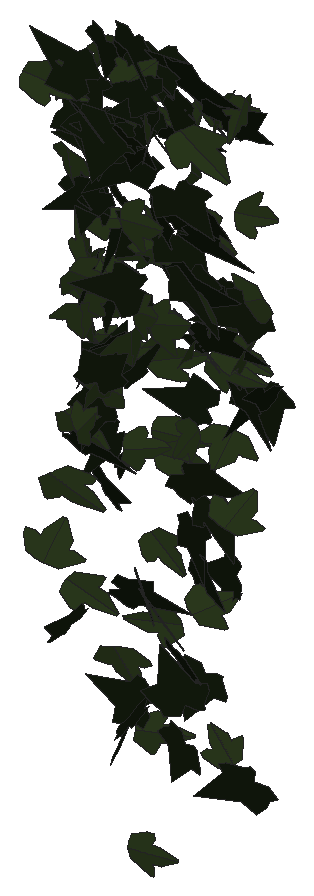
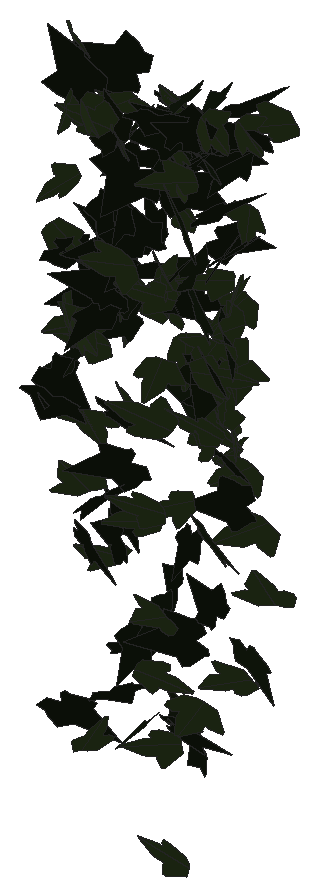
# SketchUp Ruby script. Lengths in inches.
U = 1.inch
M = Sketchup.active_model
def pt(a) = Geom::Point3d.new(a.map { |v| v * U })
def face(e, loops, mat)
  f = e.add_face(loops[0].map { |a| pt(a) })
  loops[1..].each { |l| e.add_face(l.map { |a| pt(a) }).erase! }
  f.material = f.back_material = mat if mat
  f
end
# faces: each face lists its corners as indices into pts; further lists are holes
def faces(e, pts, list, mat = nil) = list.each { |f| face(e, (f[0].is_a?(Array) ? f : [f]).map { |l| l.map { |i| pts[i] } }, mat) }
# xy, xz, yz: faces in a plane at the given z, y or x. An outline is a flat list of corners, or four numbers for a rectangle; further outlines are holes
def ring(l) = l.size == 4 ? [[l[0], l[1]], [l[2], l[1]], [l[2], l[3]], [l[0], l[3]]] : l.each_slice(2).to_a
def flat(e, list, mat, &to3) = list.each { |f| face(e, (f[0].is_a?(Array) ? f : [f]).map { |l| ring(l).map { |u, v| to3.(u, v) } }, mat) }
def xy(e, z, list, mat = nil) = flat(e, list, mat) { |x, y| [x, y, z] }
def xz(e, y, list, mat = nil) = flat(e, list, mat) { |x, z| [x, y, z] }
def yz(e, x, list, mat = nil) = flat(e, list, mat) { |y, z| [x, y, z] }
def lines(e, pts, list) = list.each { |a, b| e.add_line(pt(pts[a]), pt(pts[b])) }
# prism: a flat outline (further loops are holes) pulled along v
def prism(e, loops, v, mat = nil)
  f = face(e, loops, mat); d = Geom::Vector3d.new(v.map { |x| x * U })
  f.pushpull(f.normal.samedirection?(d) ? d.length : -d.length)
end
def box(e, o, s, mat = nil) = prism(e, [[o, [o[0] + s[0], o[1], o[2]], [o[0] + s[0], o[1] + s[1], o[2]], [o[0], o[1] + s[1], o[2]]]], [0, 0, s[2]], mat)
def at(x, y, z, deg = 0) = Geom::Transformation.translation(pt([x, y, z])) * Geom::Transformation.rotation(ORIGIN, Z_AXIS, deg.degrees)
def axes(o, x, y, z) = Geom::Transformation.new([*x, 0, *y, 0, *z, 0, *pt(o).to_a, 1])
def part(name) = M.definitions.add(name)
# library, detail: a bought-in or finely detailed component or shape, given as its bounding box
def library(name, o, s) = part(name).tap { |d| box(d.entities, o, s) }
def detail(e, o, s) = box(e.add_group.entities, o, s)
def put(e, d, t, mat = nil) = e.add_instance(d, t).tap { |i| i.material = mat if mat }
def group(e, t, mat = nil) = e.add_group.tap { |g| g.transformation = t; g.material = mat if mat }.entities
root = M.entities
M.materials.add("1026 AP 7946 SUNNY SIDE UP").color = [254, 231, 186]
M.materials.add("efeu1").color = [18, 25, 13]
M.materials.add("efeu2").color = [43, 57, 29]
c1 = part("ivyleaf_10")
p = [[0,0.5,-0.03],[-0.0625,2.02,-0.43],[-0.19,2.01,-0.46],[-0.54,1.05,-0.29],[-0.52,0.625,-0.18],[-0.83,0.76,-0.28],
  [-1.16,0.64,-0.33],[-1.15,0.33,-0.24],[-0.77,-0.39,0.02],[-0.3,-0.51,0.16],[0.04,-0.48,0.23],[-0.02,2.01,-0.4375],
  [-0.06,2.01,-0.43],[0.04,-0.49,0.23],[0.67,-0.49,0.14],[1.38,0.36,-0.2],[1.375,0.51,-0.24],[0.81,0.65,-0.19],
  [0.62,0.59,-0.15],[0.6,1.09,-0.28],[0.5,1.23,-0.31]]
faces(c1.entities,p,[[0,1,2,3,4,5,6,7,8,9,10],[11,12,0,13,14,15,16,17,18,19,20]],"efeu2")
c2 = part("ivyleaf_9")
p = [[1.54,2.16,1.25],[1.36,2.04,1.19],[-0.21,0.99,0.68],[-0.71,1.11,0.82],[-0.85,0.86,0.67],[-0.8,0.17,0.21],
  [-0.9,-0.01,0.1],[-0.67,-0.16,-0.02],[-0.08,-0.08,-0.05],[-0.03,-0.6,-0.4],[0.65,-0.88,-0.66],[0.83,-0.6,-0.49],
  [1.29,-0.42,-0.43],[1.8125,-0.07,-0.26],[1.21,0.44,0.15]]
faces(c2.entities,p,[[0,1,2,3,4,5,6,7,8,9,10,11,12,13,14]],"efeu1")
put(root,c1,axes([122.36,210.85,258.3125],[0.44754,0.08743,-0.10504],[0.13179,0.07252,0.30406],[0.16579,-0.29368,0.04184]),"1026 AP 7946 SUNNY SIDE UP")
put(root,c2,axes([123.5,210.77,262.0625],[-0.1447,-0.02833,0.30695],[0.37455,0.18207,0.09464],[-0.28534,0.25336,-0.03142]),"1026 AP 7946 SUNNY SIDE UP")
put(root,c2,axes([122.85,210.83,257.13],[-0.1457,0.26639,0.05967],[-0.04737,0.04919,-0.29],[-0.42552,-0.09669,0.01186]),"1026 AP 7946 SUNNY SIDE UP")
put(root,c1,axes([122.14,210.83,267.32],[0.11625,0.08265,0.317],[0.35672,0.20746,-0.11251],[-0.35076,0.23838,-0.00937]),"1026 AP 7946 SUNNY SIDE UP")
put(root,c1,axes([123.93,211.11,265.09],[0.11571,-0.09719,-0.31792],[0.37377,-0.19763,0.12157],[-0.34391,-0.24749,0.02517]),"1026 AP 7946 SUNNY SIDE UP")
put(root,c2,axes([125.2,210.93,256.41],[-0.38187,-0.15704,0.09928],[0.11143,0.06916,0.29773],[-0.26823,0.2523,-0.01766]),"1026 AP 7946 SUNNY SIDE UP")
put(root,c2,axes([123.44,211.15,266.71],[-0.35054,-0.24132,-0.05308],[0.08094,0.02055,-0.33746],[0.37901,-0.22758,0.02297]),"1026 AP 7946 SUNNY SIDE UP")
put(root,c2,axes([124.03,211.24,258.11],[0.15227,-0.07446,-0.29368],[0.41052,-0.11644,0.1222],[-0.21334,-0.27721,0.02553]),"1026 AP 7946 SUNNY SIDE UP")
put(root,c1,axes([122.52,211.02,259.69],[-0.32345,-0.08134,-0.24703],[0.37546,0.03869,-0.22475],[0.13038,-0.3132,0.03441]),"1026 AP 7946 SUNNY SIDE UP")
put(root,c2,axes([122.86,211.15,267.44],[-0.25822,-0.27917,0.01251],[-0.00723,0.01861,0.3335],[-0.43944,0.16374,-0.01283]),"1026 AP 7946 SUNNY SIDE UP")
put(root,c2,axes([123.82,210.875,255.03],[0.01342,0.11315,0.27549],[0.07874,0.2623,-0.11473],[-0.4488,0.0494,-0.01189]),"1026 AP 7946 SUNNY SIDE UP")
put(root,c1,axes([124.43,211.24,263.23],[0.1976,-0.12563,-0.29535],[0.35281,-0.17814,0.18116],[-0.34169,-0.25659,0.01625]),"1026 AP 7946 SUNNY SIDE UP")
put(root,c1,axes([123.99,211.28,263.28],[0.08902,-0.11725,-0.27182],[0.24144,-0.21468,0.1313],[-0.38336,-0.16243,0.01957]),"1026 AP 7946 SUNNY SIDE UP")
put(root,c2,axes([124.07,210.91,255.6],[-0.211,0.18471,-0.16679],[-0.15079,0.13174,0.23597],[0.35675,0.16493,0.0011]),"1026 AP 7946 SUNNY SIDE UP")
put(root,c2,axes([124.97,211.23,264.13],[0.11305,-0.06143,0.32606],[0.36932,-0.21269,-0.09863],[0.34808,0.24562,-0.00125]),"1026 AP 7946 SUNNY SIDE UP")
put(root,c1,axes([123,210.91,260.92],[0.09207,0.02432,-0.29656],[0.08297,0.28802,0.0378],[0.44684,-0.05849,0.05409]),"1026 AP 7946 SUNNY SIDE UP")
put(root,c1,axes([124.4,210.93,266.875],[0.03889,-0.08681,-0.30779],[-0.05694,0.29637,-0.09023],[0.48514,0.04175,0.01409]),"1026 AP 7946 SUNNY SIDE UP")
put(root,c2,axes([123.89,211.08,266.64],[0.33597,0.01275,-0.19425],[-0.29319,-0.03287,-0.22007],[-0.04917,0.28312,-0.01512]),"1026 AP 7946 SUNNY SIDE UP")
put(root,c2,axes([124.89,211.125,265.96],[-0.04417,-0.16994,-0.22851],[0.13671,0.20554,-0.17312],[0.41629,-0.08553,0.03261]),"1026 AP 7946 SUNNY SIDE UP")
put(root,c1,axes([122.85,211,263.77],[-0.14663,-0.16557,-0.25542],[0.22108,0.20354,-0.19405],[0.41199,-0.16815,0.01323]),"1026 AP 7946 SUNNY SIDE UP")
put(root,c2,axes([125.11,211.24,264.38],[0.0831,-0.31122,-0.10613],[-0.015,0.10105,-0.32453],[0.51439,0.05322,0.00768]),"1026 AP 7946 SUNNY SIDE UP")
put(root,c2,axes([126.37,211.27,255.14],[0.03124,-0.01146,-0.29775],[-0.30054,-0.21788,-0.00591],[-0.34124,0.19084,-0.02205]),"1026 AP 7946 SUNNY SIDE UP")
put(root,c2,axes([123.82,211.39,263.64],[-0.10657,-0.15746,-0.24589],[-0.14016,-0.22047,0.17528],[-0.42598,0.11193,0.00384]),"1026 AP 7946 SUNNY SIDE UP")
put(root,c1,axes([123.28,211.0625,261.76],[-0.09225,-0.18916,-0.26393],[0.11535,0.24435,-0.20259],[0.48589,-0.09392,-0.00202]),"1026 AP 7946 SUNNY SIDE UP")
put(root,c2,axes([122.73,211.17,266.76],[0.45204,-0.10754,-0.13971],[-0.20951,0.02843,-0.31547],[0.1725,0.31633,-0.01706]),"1026 AP 7946 SUNNY SIDE UP")
put(root,c2,axes([122.9375,211.44,265.14],[-0.07827,-0.05855,-0.27573],[0.01875,-0.27191,0.05748],[-0.42989,-0.0012,0.05271]),"1026 AP 7946 SUNNY SIDE UP")
put(root,c2,axes([122.9375,211.37,266.64],[-0.21194,-0.3024,-0.10247],[0.08701,0.08223,-0.34017],[0.49208,-0.14478,0.01601]),"1026 AP 7946 SUNNY SIDE UP")
put(root,c1,axes([123.97,211.29,253.01],[0.06487,-0.04016,-0.28336],[0.4051,-0.09829,0.05406],[-0.16319,-0.25995,0.02157]),"1026 AP 7946 SUNNY SIDE UP")
put(root,c2,axes([124.21,211.26,266.88],[-0.32292,0.18136,-0.04792],[0.03497,-0.04646,-0.28179],[-0.29272,-0.20561,0.0192]),"1026 AP 7946 SUNNY SIDE UP")
put(root,c1,axes([125.1,211.26,261.35],[0.29536,-0.23167,-0.08861],[-0.10604,0.05417,-0.3064],[0.37308,0.1988,-0.01694]),"1026 AP 7946 SUNNY SIDE UP")
put(root,c1,axes([125.3125,211.23,264.03],[-0.3617,0.23155,-0.00686],[-0.01783,-0.02247,-0.33548],[-0.36388,-0.22907,0.02325]),"1026 AP 7946 SUNNY SIDE UP")
put(root,c1,axes([122.625,211.24,260.82],[-0.33907,-0.02211,-0.19246],[0.29523,-0.01083,-0.22215],[0.01509,-0.28502,0.02169]),"1026 AP 7946 SUNNY SIDE UP")
put(root,c2,axes([124.75,211.5,255.2],[-0.07642,-0.23053,0.18847],[-0.03639,-0.18318,-0.24347],[0.46261,-0.05249,0.01198]),"1026 AP 7946 SUNNY SIDE UP")
put(root,c1,axes([123.79,211.26,262.76],[-0.14962,-0.32797,-0.09153],[0.04336,0.08256,-0.3513],[0.53176,-0.09901,0.0029]),"1026 AP 7946 SUNNY SIDE UP")
put(root,c2,axes([123.4375,211.5,266.36],[0.01249,-0.26469,-0.14117],[0.00871,-0.13542,0.27201],[-0.46751,-0.0096,0.00129]),"1026 AP 7946 SUNNY SIDE UP")
put(root,c2,axes([125.08,211.43,258.77],[0.06239,-0.05367,-0.2983],[0.45789,-0.03433,0.04752],[-0.06576,-0.28994,0.04781]),"1026 AP 7946 SUNNY SIDE UP")
put(root,c1,axes([125.42,211.13,258.18],[0.22467,0.03546,-0.26554],[0.29474,0.19023,0.13501],[0.28419,-0.22532,0.0699]),"1026 AP 7946 SUNNY SIDE UP")
put(root,c1,axes([122.44,211.43,267.375],[-0.00681,-0.26466,0.13888],[0.0256,-0.13634,-0.27295],[0.4674,0.00361,0.01697]),"1026 AP 7946 SUNNY SIDE UP")
put(root,c1,axes([125.06,211.25,266.93],[0.33335,0.14996,0.24914],[0.33934,0.11021,-0.26559],[-0.28989,0.30145,-0.0244]),"1026 AP 7946 SUNNY SIDE UP")
put(root,c1,axes([126,211.42,267.85],[0.33869,-0.20452,0.08017],[0.06655,-0.06984,-0.30566],[0.33825,0.21853,-0.02013]),"1026 AP 7946 SUNNY SIDE UP")
put(root,c2,axes([122.55,211.38,267.26],[-0.17257,-0.17856,-0.20495],[0.24267,0.13197,-0.21003],[0.34177,-0.18386,0.04565]),"1026 AP 7946 SUNNY SIDE UP")
put(root,c1,axes([122.48,211.32,265.73],[-0.39,0.1075,0.02896],[-0.05588,-0.01315,-0.27726],[-0.16529,-0.2492,0.02539]),"1026 AP 7946 SUNNY SIDE UP")
put(root,c2,axes([122.93,211.5,261.14],[-0.367,-0.02217,-0.17858],[0.27446,-0.03899,-0.23737],[-0.00891,-0.28803,0.04415]),"1026 AP 7946 SUNNY SIDE UP")
put(root,c1,axes([122.78,211.28,263.99],[-0.08198,0.29231,-0.12152],[-0.04152,0.11678,0.30652],[0.49488,0.05822,0.00559]),"1026 AP 7946 SUNNY SIDE UP")
put(root,c1,axes([125.08,211.31,263.0625],[0.03891,-0.25745,-0.16723],[-0.03159,0.15966,-0.26548],[0.4763,0.03162,-0.00395]),"1026 AP 7946 SUNNY SIDE UP")
put(root,c2,axes([122.64,211.6,265.04],[-0.08327,-0.27179,0.1015],[-0.01949,-0.09951,-0.28576],[0.45498,-0.05401,0.00633]),"1026 AP 7946 SUNNY SIDE UP")
put(root,c2,axes([126.14,211.62,263.92],[-0.03296,-0.12863,-0.28079],[-0.08965,-0.26584,0.13257],[-0.46429,0.06047,-0.00567]),"1026 AP 7946 SUNNY SIDE UP")
put(root,c1,axes([122.61,211.41,262.8],[-0.2696,-0.23067,-0.02654],[0.05051,0.0065,-0.2952],[0.36122,-0.17307,0.02147]),"1026 AP 7946 SUNNY SIDE UP")
put(root,c2,axes([125.24,211.29,263.28],[0.43908,0.06053,0.164],[0.25525,-0.00426,-0.29232],[-0.07936,0.32123,-0.03284]),"1026 AP 7946 SUNNY SIDE UP")
put(root,c1,axes([123.36,211.375,261.52],[-0.07389,0.03511,0.30084],[-0.46204,0.00121,-0.04889],[-0.01067,-0.29558,0.03378]),"1026 AP 7946 SUNNY SIDE UP")
put(root,c1,axes([123.3125,211.39,262.24],[0.30216,-0.20761,-0.15265],[-0.17122,0.09936,-0.29063],[0.36149,0.2206,-0.01006]),"1026 AP 7946 SUNNY SIDE UP")
put(root,c2,axes([123.65,211.6,265.96],[-0.00051,0.04662,-0.32889],[-0.02062,-0.31925,-0.04985],[-0.5073,0.01293,0.00236]),"1026 AP 7946 SUNNY SIDE UP")
put(root,c2,axes([124.05,211.41,257.73],[0.38203,-0.14935,-0.06709],[-0.1013,0.01768,-0.2931],[0.23474,0.2507,-0.0173]),"1026 AP 7946 SUNNY SIDE UP")
put(root,c2,axes([123.23,211.3,261.99],[-0.22088,-0.05762,0.24063],[0.31047,0.12759,0.15528],[-0.21701,0.24118,-0.02277]),"1026 AP 7946 SUNNY SIDE UP")
put(root,c2,axes([123.28,211.33,266.4],[-0.1527,0.24814,0.06992],[0.0119,-0.06826,0.27353],[0.40376,0.09586,0.01838]),"1026 AP 7946 SUNNY SIDE UP")
put(root,c2,axes([124.7,211.37,256.98],[0.38008,-0.06796,-0.15877],[-0.23759,0.03009,-0.25829],[0.11577,0.28488,-0.00882]),"1026 AP 7946 SUNNY SIDE UP")
put(root,c1,axes([122.64,211.49,263.0625],[-0.3081,0.04828,0.2401],[0.3668,-0.01919,0.20626],[0.07216,0.30367,-0.02331]),"1026 AP 7946 SUNNY SIDE UP")
put(root,c2,axes([124.11,211.65,264.89],[0.01182,-0.04025,0.30005],[0.08881,-0.28596,-0.04385],[0.45408,0.05698,0.00077]),"1026 AP 7946 SUNNY SIDE UP")
put(root,c2,axes([122.45,211.47,260.3],[0.37466,-0.0583,0.15651],[0.21841,-0.06855,-0.2514],[0.13421,0.27433,-0.02778]),"1026 AP 7946 SUNNY SIDE UP")
put(root,c2,axes([123.88,211.71,266.96],[0.05519,-0.20113,-0.20108],[0.06269,-0.18997,0.20917],[-0.43496,-0.0529,0.00463]),"1026 AP 7946 SUNNY SIDE UP")
put(root,c2,axes([124.01,211.48,267.34],[-0.32373,0.12378,0.14307],[-0.21708,0.03563,-0.2446],[-0.19483,-0.24538,0.03482]),"1026 AP 7946 SUNNY SIDE UP")
put(root,c2,axes([124.84,211.625,259.39],[-0.20036,-0.01193,-0.30965],[0.46975,-0.04258,-0.12901],[-0.05443,-0.32361,0.02647]),"1026 AP 7946 SUNNY SIDE UP")
put(root,c2,axes([123.85,211.49,255.66],[-0.28605,-0.06572,-0.2285],[-0.347,-0.03376,0.1969],[-0.10722,0.28458,-0.02763]),"1026 AP 7946 SUNNY SIDE UP")
put(root,c2,axes([123.67,211.35,261.875],[-0.16479,0.29427,-0.01344],[0.00696,0.01719,0.32174],[0.46324,0.10442,-0.00961]),"1026 AP 7946 SUNNY SIDE UP")
put(root,c1,axes([122.68,211.45,261.82],[0.13429,-0.24556,-0.15908],[-0.0404,0.15248,-0.26596],[0.45316,0.08637,0.02343]),"1026 AP 7946 SUNNY SIDE UP")
put(root,c2,axes([123.22,211.36,262.41],[0.13332,0.26789,0.07083],[0.04047,0.06236,-0.28905],[-0.43241,0.08843,-0.00521]),"1026 AP 7946 SUNNY SIDE UP")
put(root,c1,axes([123.84,211.77,264.24],[-0.01504,0.01408,0.30357],[-0.01654,-0.29458,0.01243],[0.46346,-0.01006,0.0103]),"1026 AP 7946 SUNNY SIDE UP")
put(root,c2,axes([123.57,211.8125,264.43],[-0.11084,-0.17552,0.22986],[-0.11119,-0.21286,-0.19589],[0.43359,-0.09945,0.00853]),"1026 AP 7946 SUNNY SIDE UP")
put(root,c2,axes([124.61,211.66,267.79],[0.26297,-0.11977,0.27887],[0.32838,-0.17371,-0.21258],[0.33124,0.26729,-0.01065]),"1026 AP 7946 SUNNY SIDE UP")
put(root,c1,axes([124.02,211.43,255.25],[-0.02033,-0.05276,-0.29874],[0.388,0.15626,-0.03975],[0.25261,-0.24426,0.03702]),"1026 AP 7946 SUNNY SIDE UP")
put(root,c1,axes([126.22,211.58,264.18],[-0.28623,0.03692,0.25454],[-0.39155,-0.04805,-0.18204],[0.02723,-0.30294,0.05805]),"1026 AP 7946 SUNNY SIDE UP")
put(root,c2,axes([122.84,211.38,263.51],[-0.09603,0.00363,-0.34781],[-0.43908,0.19237,0.05529],[0.29851,0.28412,-0.03057]),"1026 AP 7946 SUNNY SIDE UP")
put(root,c2,axes([122.83,211.82,267.8],[-0.00171,-0.21539,0.18451],[0.01316,-0.18028,-0.22283],[0.44152,0.00454,0.00736]),"1026 AP 7946 SUNNY SIDE UP")
put(root,c1,axes([122.66,211.39,263.57],[0.05404,-0.06648,0.31491],[-0.11813,0.29716,0.07693],[-0.4781,-0.08094,0.01659]),"1026 AP 7946 SUNNY SIDE UP")
put(root,c2,axes([124.6,211.625,263.2],[0.37983,-0.1714,-0.02992],[-0.05722,-0.00293,-0.3042],[0.26704,0.24317,-0.02263]),"1026 AP 7946 SUNNY SIDE UP")
put(root,c2,axes([122.78,211.84,264.75],[-0.1064,-0.03868,0.28712],[-0.14803,-0.26725,-0.06327],[0.4173,-0.10466,0.05076]),"1026 AP 7946 SUNNY SIDE UP")
put(root,c1,axes([123.44,211.6,267.33],[0.3956,-0.04006,-0.16192],[0.25339,0.03267,0.25773],[-0.02568,-0.29472,0.0488]),"1026 AP 7946 SUNNY SIDE UP")
put(root,c2,axes([125.43,211.72,267.25],[0.52344,0.02891,-0.07935],[0.11416,0.04921,0.34184],[0.06136,-0.33816,0.04093]),"1026 AP 7946 SUNNY SIDE UP")
put(root,c2,axes([124.71,211.86,263.35],[0.293,-0.22667,-0.05803],[0.0774,-0.03065,0.30153],[-0.35852,-0.19187,0.01767]),"1026 AP 7946 SUNNY SIDE UP")
put(root,c2,axes([124.79,211.55,260.33],[0.08515,0.01588,-0.28775],[0.17167,0.26084,0.0386],[0.40518,-0.11386,0.04411]),"1026 AP 7946 SUNNY SIDE UP")
put(root,c1,axes([123.23,211.68,256.31],[-0.4294,-0.0414,-0.10382],[0.16245,-0.01405,-0.2832],[0.05331,-0.29067,0.02674]),"1026 AP 7946 SUNNY SIDE UP")
put(root,c2,axes([122.88,211.93,265.8],[-0.02225,-0.27319,-0.16484],[-0.01925,-0.15803,0.28086],[-0.49622,0.01838,-0.00351]),"1026 AP 7946 SUNNY SIDE UP")
put(root,c1,axes([122.5625,211.76,262.07],[-0.35585,0.16669,0.06395],[0.09247,-0.02307,0.28896],[0.26342,0.23328,-0.01505]),"1026 AP 7946 SUNNY SIDE UP")
put(root,c2,axes([125.7,211.86,262.06],[0.21444,-0.26316,0.05687],[0.02256,-0.05636,-0.30538],[0.42268,0.13651,-0.01255]),"1026 AP 7946 SUNNY SIDE UP")
put(root,c2,axes([125.71,211.64,258.7],[-0.09132,-0.01487,-0.30703],[-0.466,0.0376,0.0578],[0.05366,0.30122,-0.02058]),"1026 AP 7946 SUNNY SIDE UP")
put(root,c1,axes([125.28,211.78,262.51],[-0.05763,-0.05727,-0.30266],[0.46634,-0.04454,-0.02947],[-0.05975,-0.29237,0.06196]),"1026 AP 7946 SUNNY SIDE UP")
put(root,c2,axes([125.12,211.85,259.71],[0.04608,-0.28352,-0.07825],[-0.01687,0.07363,-0.29319],[0.46058,0.03106,-0.00291]),"1026 AP 7946 SUNNY SIDE UP")
put(root,c1,axes([125.87,211.78,263.02],[0.09196,-0.31035,-0.06656],[-0.00338,0.06352,-0.32483],[0.49788,0.05775,0.01009]),"1026 AP 7946 SUNNY SIDE UP")
put(root,c2,axes([123.32,211.69,257.57],[0.35133,0.03857,0.19067],[0.29487,-0.01156,-0.23108],[-0.035,0.28977,-0.03287]),"1026 AP 7946 SUNNY SIDE UP")
put(root,c1,axes([122.72,211.66,264.52],[0.05206,-0.0526,-0.29029],[0.37306,0.1637,-0.0018],[0.25212,-0.23137,0.06261]),"1026 AP 7946 SUNNY SIDE UP")
put(root,c1,axes([125.42,211.86,261.14],[0.43953,0.06615,-0.06952],[-0.09586,-0.03629,-0.29536],[-0.11408,0.28535,-0.01966]),"1026 AP 7946 SUNNY SIDE UP")
put(root,c1,axes([122.99,211.69,261.37],[0.13974,-0.19828,0.19526],[-0.10402,0.17908,0.22467],[-0.41984,-0.11036,0.00932]),"1026 AP 7946 SUNNY SIDE UP")
put(root,c2,axes([123.46,211.8,266.76],[0.38894,-0.14883,-0.06474],[-0.09715,0.01738,-0.2968],[0.23417,0.25441,-0.01559]),"1026 AP 7946 SUNNY SIDE UP")
put(root,c1,axes([125.57,211.71,259.69],[0.33749,0.12593,-0.17346],[0.20634,0.10906,0.25592],[0.25946,-0.25053,0.02211]),"1026 AP 7946 SUNNY SIDE UP")
put(root,c1,axes([122.87,211.93,262.8125],[0.06218,0.0561,0.31201],[-0.40238,-0.16338,0.06471],[0.26866,-0.25769,0.02471]),"1026 AP 7946 SUNNY SIDE UP")
put(root,c1,axes([122.26,211.76,257.23],[0.17787,0.11629,0.24861],[0.31817,0.13348,-0.16365],[-0.27459,0.22999,-0.02858]),"1026 AP 7946 SUNNY SIDE UP")
put(root,c2,axes([124.74,212.04,256.28],[-0.22359,-0.24202,0.04378],[-0.01604,-0.04483,-0.28909],[0.38642,-0.1419,0.01333]),"1026 AP 7946 SUNNY SIDE UP")
put(root,c1,axes([124.74,211.69,266.06],[-0.00088,-0.22341,-0.28259],[-0.00415,0.27303,-0.22855],[0.55472,0.00169,-0.00216]),"1026 AP 7946 SUNNY SIDE UP")
put(root,c2,axes([124.88,211.86,263.7],[0.16414,0.01683,-0.28851],[0.38658,0.13869,0.10377],[0.21287,-0.26485,0.03403]),"1026 AP 7946 SUNNY SIDE UP")
put(root,c2,axes([124.19,211.91,264.82],[0.4202,0.12014,0.03029],[-0.06258,0.01896,0.29998],[0.18387,-0.2681,0.03289]),"1026 AP 7946 SUNNY SIDE UP")
put(root,c1,axes([123.63,211.9,266.85],[0.34752,-0.18568,-0.10151],[-0.12159,0.05949,-0.297],[0.30652,0.23412,-0.00272]),"1026 AP 7946 SUNNY SIDE UP")
put(root,c2,axes([122.96,212.09,264.75],[0.12573,-0.2204,0.18008],[0.07041,-0.17076,-0.24217],[0.43793,0.09073,-0.01277]),"1026 AP 7946 SUNNY SIDE UP")
put(root,c2,axes([122.76,212.02,263.11],[-0.27127,0.00912,-0.24331],[0.36345,-0.05482,-0.17641],[-0.07795,-0.28733,0.02419]),"1026 AP 7946 SUNNY SIDE UP")
put(root,c1,axes([125.34,211.91,255.01],[0.10341,0.2716,0.0628],[-0.03966,-0.05497,0.28733],[0.43536,-0.06952,0.01126]),"1026 AP 7946 SUNNY SIDE UP")
put(root,c2,axes([123.21,212.09,267.88],[0.0604,-0.27179,0.10058],[0.02768,-0.09766,-0.28333],[0.45409,0.04211,0.00389]),"1026 AP 7946 SUNNY SIDE UP")
put(root,c2,axes([124.25,211.92,267.08],[0.2453,-0.23787,-0.12001],[-0.10818,0.09254,-0.29243],[0.40121,0.17038,-0.00548]),"1026 AP 7946 SUNNY SIDE UP")
put(root,c1,axes([125.45,211.8,262.86],[0.16091,0.1119,0.26968],[0.30209,0.17722,-0.15476],[-0.32911,0.21739,-0.0102]),"1026 AP 7946 SUNNY SIDE UP")
put(root,c1,axes([122.7,212.07,267.63],[-0.00409,-0.27505,0.15013],[0.00358,-0.14731,-0.28421],[0.49059,-0.00122,0.00333]),"1026 AP 7946 SUNNY SIDE UP")
put(root,c1,axes([122.69,211.92,263.42],[0.35171,0.15343,0.1003],[0.14311,0.03746,-0.2785],[-0.24646,0.2407,-0.01858]),"1026 AP 7946 SUNNY SIDE UP")
put(root,c2,axes([124.77,211.89,265.25],[0.41254,-0.01671,-0.18388],[-0.2807,0.00269,-0.27072],[0.02411,0.31726,-0.00553]),"1026 AP 7946 SUNNY SIDE UP")
put(root,c1,axes([123.34,211.98,266.2],[0.2665,-0.23731,0.02005],[0.00413,0.0274,0.30001],[-0.37456,-0.16855,0.01757]),"1026 AP 7946 SUNNY SIDE UP")
put(root,c2,axes([124.79,211.97,261.45],[-0.28142,0.12073,0.20371],[-0.28284,0.0837,-0.22064],[-0.22813,-0.2527,0.02226]),"1026 AP 7946 SUNNY SIDE UP")
put(root,c2,axes([124.1875,212.01,264.45],[-0.02559,-0.21081,-0.19876],[0.0919,0.1855,-0.21413],[0.43855,-0.05117,0.03327]),"1026 AP 7946 SUNNY SIDE UP")
put(root,c2,axes([124.54,211.99,264.61],[0.40092,-0.03593,0.12962],[0.192,-0.03494,-0.26497],[0.0748,0.28226,-0.0146]),"1026 AP 7946 SUNNY SIDE UP")
put(root,c2,axes([122.89,212.17,264.21],[-0.29343,0.08015,-0.25156],[0.32717,-0.13096,-0.20847],[-0.23836,-0.27842,0.02352]),"1026 AP 7946 SUNNY SIDE UP")
put(root,c1,axes([123.35,211.88,260.21],[0.0085,-0.04458,-0.30208],[0.29881,0.22536,-0.0304],[0.35755,-0.18728,0.03258]),"1026 AP 7946 SUNNY SIDE UP")
put(root,c1,axes([125.28,212.23,263.04],[0.09964,-0.2894,0.15743],[0.05289,-0.15075,-0.30608],[0.51308,0.07174,0.00098]),"1026 AP 7946 SUNNY SIDE UP")
put(root,c1,axes([122.67,212.04,261.82],[0.18963,-0.06082,-0.2695],[0.42102,0.01006,0.12498],[-0.02538,-0.28757,0.05962]),"1026 AP 7946 SUNNY SIDE UP")
put(root,c2,axes([125.85,212.2,261.97],[-0.1312,0.17966,-0.27727],[0.14874,-0.25336,-0.20516],[-0.488,-0.12552,0.01202]),"1026 AP 7946 SUNNY SIDE UP")
put(root,c1,axes([123.92,212.14,256.95],[0.12628,-0.0224,-0.27618],[-0.42279,-0.0041,-0.08269],[0.00391,0.2797,-0.02168]),"1026 AP 7946 SUNNY SIDE UP")
put(root,c1,axes([123.78,211.95,264.38],[0.13912,-0.04151,0.2884],[-0.34565,0.17504,0.09925],[-0.28085,-0.23599,0.02071]),"1026 AP 7946 SUNNY SIDE UP")
put(root,c1,axes([123.75,212.05,262.7],[-0.23513,-0.22999,-0.12338],[0.12819,0.08796,-0.28143],[0.38606,-0.16928,0.0183]),"1026 AP 7946 SUNNY SIDE UP")
put(root,c1,axes([125.75,211.89,265.5],[0.00255,0.11648,0.29046],[0.01452,0.28114,-0.11834],[-0.4785,0.00915,-0.00204]),"1026 AP 7946 SUNNY SIDE UP")
put(root,c2,axes([123.35,212.17,267.27],[0.36875,-0.14744,0.11135],[0.12178,-0.08062,-0.28467],[0.26125,0.24569,-0.02448]),"1026 AP 7946 SUNNY SIDE UP")
put(root,c2,axes([122.68,212.23,260.07],[-0.40349,0.09682,-0.17196],[0.221,-0.09784,-0.28071],[-0.209,-0.29038,0.03516]),"1026 AP 7946 SUNNY SIDE UP")
put(root,c1,axes([124.48,212.23,266.89],[0.24986,-0.23684,0.05357],[0.02972,-0.0515,-0.29382],[0.38058,0.15951,-0.01223]),"1026 AP 7946 SUNNY SIDE UP")
put(root,c1,axes([123.64,212.07,264.06],[0.12448,-0.00713,-0.29425],[0.42195,0.10349,0.07458],[0.15406,-0.2777,0.03349]),"1026 AP 7946 SUNNY SIDE UP")
put(root,c2,axes([124.4,212.35,266.93],[0.35595,-0.13033,-0.15465],[0.22801,-0.04574,0.26723],[-0.21254,-0.26733,0.02769]),"1026 AP 7946 SUNNY SIDE UP")
put(root,c2,axes([122.91,212.17,267.38],[0.10959,-0.01885,0.29124],[0.42441,-0.0845,-0.07482],[0.13606,0.27875,-0.0012]),"1026 AP 7946 SUNNY SIDE UP")
put(root,c1,axes([125.02,212.33,267.25],[0.08286,-0.28138,0.10151],[0.031,-0.09818,-0.29549],[0.4686,0.05625,0.0016]),"1026 AP 7946 SUNNY SIDE UP")
put(root,c2,axes([123.54,212.32,267.61],[-0.22749,-0.21181,-0.15136],[0.15798,0.10733,-0.26286],[0.37211,-0.17506,0.01906]),"1026 AP 7946 SUNNY SIDE UP")
put(root,c2,axes([124.09,212.21,266.36],[0.48326,0.08081,-0.05896],[-0.07513,-0.04413,-0.32617],[-0.13686,0.30958,-0.02914]),"1026 AP 7946 SUNNY SIDE UP")
put(root,c1,axes([123.14,212.16,266.47],[0.05452,0.06255,0.29458],[0.28842,0.21929,-0.07114],[-0.35797,0.18621,-0.01246]),"1026 AP 7946 SUNNY SIDE UP")
put(root,c1,axes([124.77,212.23,266.98],[-0.1676,-0.04777,0.27446],[0.33569,0.16163,0.11868],[-0.26229,0.2374,-0.02349]),"1026 AP 7946 SUNNY SIDE UP")
put(root,c1,axes([123.46,212.37,258.26],[0.27361,0.03862,0.22245],[0.34072,0.01079,-0.182],[-0.05143,0.27694,-0.02228]),"1026 AP 7946 SUNNY SIDE UP")
put(root,c2,axes([122.2,212.53,258.83],[0.06468,-0.08495,0.26779],[0.1772,-0.23477,-0.09861],[0.39258,0.11997,0.00039]),"1026 AP 7946 SUNNY SIDE UP")
put(root,c1,axes([124.22,212.43,264.64],[-0.22629,0.02676,-0.30678],[0.42908,-0.12372,-0.14796],[-0.19271,-0.30688,0.03079]),"1026 AP 7946 SUNNY SIDE UP")
put(root,c1,axes([123.59,212.26,261.78],[-0.18283,-0.08192,0.30184],[0.33264,0.20433,0.14631],[-0.34477,0.24059,-0.0189]),"1026 AP 7946 SUNNY SIDE UP")
put(root,c1,axes([125.46,212.2,267.15],[0.00129,-0.14756,-0.26246],[0.02913,0.25345,-0.15018],[0.46088,-0.01561,0.01023]),"1026 AP 7946 SUNNY SIDE UP")
put(root,c2,axes([122.96,212.21,259.87],[-0.0072,-0.018,-0.28351],[-0.26153,0.2196,-0.01067],[0.3457,0.16575,-0.01398]),"1026 AP 7946 SUNNY SIDE UP")
put(root,c2,axes([124.8,212.31,263.5],[0.03768,-0.14634,-0.25032],[-0.08135,0.23665,-0.15122],[0.43738,0.05662,-0.00656]),"1026 AP 7946 SUNNY SIDE UP")
put(root,c1,axes([123.74,212.34,259.97],[0.04538,0.04987,0.28384],[0.27647,0.21196,-0.05732],[-0.34207,0.17793,-0.00867]),"1026 AP 7946 SUNNY SIDE UP")
put(root,c2,axes([122.77,212.49,265.58],[-0.08974,0.26051,0.19968],[-0.00483,-0.19574,0.27102],[0.50916,0.04406,0.03776]),"1026 AP 7946 SUNNY SIDE UP")
put(root,c2,axes([125.54,212.6,261.76],[-0.26742,-0.12684,-0.20456],[0.28655,0.08302,-0.21573],[0.23332,-0.24733,0.0305]),"1026 AP 7946 SUNNY SIDE UP")
put(root,c1,axes([123.53,212.51,260.3],[0.00484,-0.03857,-0.28776],[0.44295,-0.00514,0.0039],[-0.00883,-0.27908,0.03803]),"1026 AP 7946 SUNNY SIDE UP")
